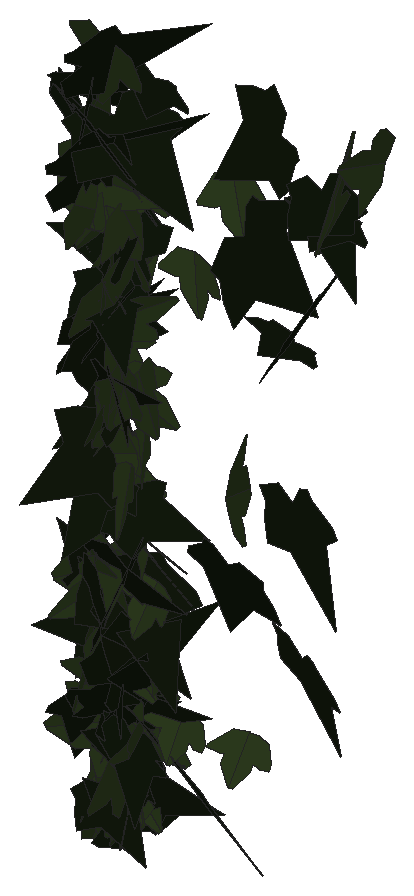
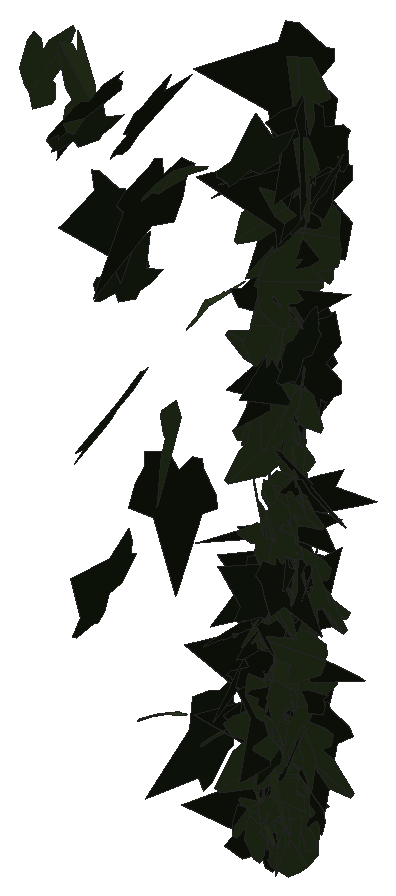
# SketchUp Ruby script. Lengths in inches.
U = 1.inch
M = Sketchup.active_model
def pt(a) = Geom::Point3d.new(a.map { |v| v * U })
def face(e, loops, mat)
  f = e.add_face(loops[0].map { |a| pt(a) })
  loops[1..].each { |l| e.add_face(l.map { |a| pt(a) }).erase! }
  f.material = f.back_material = mat if mat
  f
end
# faces: each face lists its corners as indices into pts; further lists are holes
def faces(e, pts, list, mat = nil) = list.each { |f| face(e, (f[0].is_a?(Array) ? f : [f]).map { |l| l.map { |i| pts[i] } }, mat) }
# xy, xz, yz: faces in a plane at the given z, y or x. An outline is a flat list of corners, or four numbers for a rectangle; further outlines are holes
def ring(l) = l.size == 4 ? [[l[0], l[1]], [l[2], l[1]], [l[2], l[3]], [l[0], l[3]]] : l.each_slice(2).to_a
def flat(e, list, mat, &to3) = list.each { |f| face(e, (f[0].is_a?(Array) ? f : [f]).map { |l| ring(l).map { |u, v| to3.(u, v) } }, mat) }
def xy(e, z, list, mat = nil) = flat(e, list, mat) { |x, y| [x, y, z] }
def xz(e, y, list, mat = nil) = flat(e, list, mat) { |x, z| [x, y, z] }
def yz(e, x, list, mat = nil) = flat(e, list, mat) { |y, z| [x, y, z] }
def lines(e, pts, list) = list.each { |a, b| e.add_line(pt(pts[a]), pt(pts[b])) }
# prism: a flat outline (further loops are holes) pulled along v
def prism(e, loops, v, mat = nil)
  f = face(e, loops, mat); d = Geom::Vector3d.new(v.map { |x| x * U })
  f.pushpull(f.normal.samedirection?(d) ? d.length : -d.length)
end
def box(e, o, s, mat = nil) = prism(e, [[o, [o[0] + s[0], o[1], o[2]], [o[0] + s[0], o[1] + s[1], o[2]], [o[0], o[1] + s[1], o[2]]]], [0, 0, s[2]], mat)
def at(x, y, z, deg = 0) = Geom::Transformation.translation(pt([x, y, z])) * Geom::Transformation.rotation(ORIGIN, Z_AXIS, deg.degrees)
def axes(o, x, y, z) = Geom::Transformation.new([*x, 0, *y, 0, *z, 0, *pt(o).to_a, 1])
def part(name) = M.definitions.add(name)
# library, detail: a bought-in or finely detailed component or shape, given as its bounding box
def library(name, o, s) = part(name).tap { |d| box(d.entities, o, s) }
def detail(e, o, s) = box(e.add_group.entities, o, s)
def put(e, d, t, mat = nil) = e.add_instance(d, t).tap { |i| i.material = mat if mat }
def group(e, t, mat = nil) = e.add_group.tap { |g| g.transformation = t; g.material = mat if mat }.entities
root = M.entities
M.materials.add("efeu1").color = [18, 25, 13]
M.materials.add("efeu2").color = [43, 57, 29]
c1 = part("ivyleaf_10")
p = [[0,0.5,-0.03],[-0.0625,2.02,-0.43],[-0.19,2.01,-0.46],[-0.54,1.05,-0.29],[-0.52,0.625,-0.18],[-0.83,0.76,-0.28],
  [-1.16,0.64,-0.33],[-1.15,0.33,-0.24],[-0.77,-0.39,0.02],[-0.3,-0.51,0.16],[0.04,-0.48,0.23],[-0.02,2.01,-0.4375],
  [-0.06,2.01,-0.43],[0.04,-0.49,0.23],[0.67,-0.49,0.14],[1.38,0.36,-0.2],[1.375,0.51,-0.24],[0.81,0.65,-0.19],
  [0.62,0.59,-0.15],[0.6,1.09,-0.28],[0.5,1.23,-0.31]]
faces(c1.entities,p,[[0,1,2,3,4,5,6,7,8,9,10],[11,12,0,13,14,15,16,17,18,19,20]],"efeu2")
c2 = part("ivyleaf_9")
p = [[1.54,2.16,1.25],[1.36,2.04,1.19],[-0.21,0.99,0.68],[-0.71,1.11,0.82],[-0.85,0.86,0.67],[-0.8,0.17,0.21],
  [-0.9,-0.01,0.1],[-0.67,-0.16,-0.02],[-0.08,-0.08,-0.05],[-0.03,-0.6,-0.4],[0.65,-0.88,-0.66],[0.83,-0.6,-0.49],
  [1.29,-0.42,-0.43],[1.8125,-0.07,-0.26],[1.21,0.44,0.15]]
faces(c2.entities,p,[[0,1,2,3,4,5,6,7,8,9,10,11,12,13,14]],"efeu1")
put(root,c1,axes([585.83,126.8,191.39],[0.53588,-0.21194,-0.8665],[-0.80039,0.33208,-0.57622],[0.39386,0.96318,0.008]))
put(root,c1,axes([585.97,126.76,206.64],[-0.97546,0.08442,0.38421],[-0.38156,0.04674,-0.97903],[-0.09566,-1.04736,-0.01272]))
put(root,c1,axes([585.76,127.4375,190.76],[0.22117,0.36477,-0.87026],[-0.59752,-0.63767,-0.41913],[-0.73033,0.63218,0.07937]))
put(root,c2,axes([585.8,126.18,206.35],[0.1962,0.8705,-0.7375],[0.14249,0.72377,0.8922],[1.13197,-0.24198,0.01552]))
put(root,c2,axes([585.68,127.14,191.08],[0.52201,-0.39717,0.77495],[0.6744,-0.3872,-0.65272],[0.55089,0.85036,0.06474]))
put(root,c2,axes([585.32,126.58,204.45],[1.26759,-0.16301,-0.50833],[-0.49862,0.10623,-1.27744],[0.19066,1.36158,0.0388]))
put(root,c2,axes([586.25,127.48,186.12],[0.08288,-0.84438,0.23188],[0.09411,-0.22298,-0.8456],[0.87057,0.1045,0.06934]))
put(root,c1,axes([586.25,127.21,193.9],[0.60781,-0.3979,0.23932],[0.19688,-0.13618,-0.72645],[0.42052,0.63888,-0.00579]))
put(root,c2,axes([590.04,126.7,192.86],[0.72145,0.31331,-0.76378],[-0.73389,-0.2211,-0.78392],[-0.37805,1.02712,0.06424]))
put(root,c2,axes([585.72,127.19,199.44],[0.00525,-0.77499,-0.26252],[0.01443,0.26258,-0.77485],[0.81812,0.00034,0.01535]))
put(root,c2,axes([586.1,127.62,185.38],[0.5714,-0.79133,-0.15741],[0.10342,-0.11947,0.97597],[-0.80018,-0.58053,0.01373]))
put(root,c2,axes([584.45,127.69,203.85],[0.19177,-0.77719,0.6517],[0.16789,-0.62977,-0.80044],[1.00027,0.2547,0.00941]))
put(root,c1,axes([585.67,127.17,188.01],[-0.73952,-0.35537,-0.0641],[-0.05305,-0.03758,0.8204],[-0.35719,0.74134,0.01087]))
put(root,c2,axes([585.59,127.45,193.39],[-0.59969,-0.49951,0.03874],[-0.02928,-0.02537,-0.78047],[0.50015,-0.60041,0.00076]))
put(root,c2,axes([585.74,127.01,184.65],[-0.2181,-0.29266,-0.67092],[0.47467,0.47636,-0.3621],[0.5572,-0.52036,0.04586]))
put(root,c1,axes([585.95,126.73,199.6],[-0.18116,-0.87389,-0.5283],[0.13264,0.51186,-0.89219],[1.01252,-0.22341,0.02236]))
put(root,c2,axes([585.31,127.78,194.21],[-0.59416,-0.54054,0.56045],[-0.38707,-0.40667,-0.80257],[0.67562,-0.70834,0.03308]))
put(root,c2,axes([585.73,127.15,186.94],[0.8681,0.5207,0.17599],[-0.15252,-0.08785,1.01228],[0.52805,-0.88139,0.00307]))
put(root,c2,axes([585.875,127.08,202.96],[0.24927,-0.25277,0.76845],[-0.58189,0.50257,0.35407],[-0.56197,-0.63251,-0.02576]))
put(root,c2,axes([585.68,127.51,196.34],[0.26604,-0.07043,-0.74306],[0.7081,-0.22562,0.27491],[-0.23601,-0.75632,-0.01281]))
put(root,c2,axes([585.64,127.28,190.48],[0.40618,-0.07857,0.7094],[-0.68976,0.1666,0.41338],[-0.18346,-0.8003,0.01641]))
put(root,c2,axes([585.38,127.25,196.36],[0.28354,-0.28326,0.65236],[0.60154,-0.27915,-0.38266],[0.37942,0.65425,0.11917]))
put(root,c1,axes([586.39,127.03,185.82],[0.12881,-1.16578,-0.32263],[0.12747,0.33573,-1.16222],[1.20286,0.08926,0.15772]))
put(root,c1,axes([586.01,127.07,196.53],[-0.72562,0.02431,0.27132],[-0.27156,-0.00338,-0.72594],[-0.02159,-0.77469,0.01168]))
put(root,c2,axes([585.23,126.3,202.9],[0.22606,1.05829,-0.73534],[0.08914,0.73194,1.0808],[1.2856,-0.23685,0.05436]))
put(root,c2,axes([585.64,127.29,189.57],[0.0896,0.87466,0.70671],[-0.07755,-0.70246,0.87923],[1.12181,-0.11842,0.00433]))
put(root,c1,axes([585.53,126.99,191.18],[-0.88666,0.21945,0.46734],[-0.45458,0.10852,-0.91341],[-0.24479,-0.99639,0.00345]))
put(root,c1,axes([586.01,127.17,197.09],[-0.62727,0.01494,0.45907],[-0.45909,-0.04439,-0.62586],[0.01418,-0.77605,0.04464]))
put(root,c2,axes([585.42,126.95,191.3125],[0.67678,-0.43776,-0.65378],[-0.55675,0.3429,-0.80594],[0.55596,0.87629,-0.01123]))
put(root,c2,axes([585.29,127.13,187.16],[0.25446,0.66269,-0.48536],[-0.16703,-0.45575,-0.70983],[-0.80425,0.30432,-0.00614]))
put(root,c2,axes([591.52,127.5625,194.73],[0.52714,-1.01866,0.01643],[0.00752,-0.01461,-1.14698],[1.01877,0.52719,-0.00003]))
put(root,c1,axes([585.21,126.77,201.78],[-0.12539,-0.48745,-0.72412],[0.24432,0.68272,-0.50188],[0.83802,-0.27198,0.03798]))
put(root,c2,axes([585.86,127.37,204.24],[0.33074,-1.05423,-0.43486],[0.41693,0.53322,-0.97558],[1.06145,0.11905,0.5187]))
put(root,c2,axes([588.22,127.22,185.86],[1.02842,-0.44574,-0.06664],[-0.0621,0.02431,-1.12086],[0.4464,1.03029,-0.00239]))
put(root,c1,axes([585.85,127.1875,188.89],[0.54081,0.29658,0.61881],[0.55533,0.27369,-0.61649],[-0.40311,0.77492,-0.0191]))
put(root,c1,axes([593.01,127.03,203.67],[0.62587,-0.96913,0.5274],[-0.28236,0.44547,1.15365],[-1.0666,-0.68661,0.00407]))
put(root,c1,axes([584.82,128.01,188.22],[-0.02958,0.51375,-0.97381],[0.08461,-0.97022,-0.51442],[-1.09776,-0.08863,-0.01341]))
put(root,c1,axes([584.8,127.11,202.35],[0.0716,-0.05686,1.17592],[1.06714,0.50069,-0.04077],[-0.49722,1.06641,0.08184]))
put(root,c1,axes([585.37,127.3,186.43],[0.44016,-0.14131,-0.89437],[-0.85731,0.25494,-0.4622],[0.29134,0.96366,-0.00887]))
put(root,c1,axes([585.79,127.25,183.84],[0.86466,-0.04091,0.48702],[-0.48644,0.02381,0.86562],[-0.04733,-0.99209,0.00069]))
put(root,c2,axes([585.25,126.47,197.9],[0.32694,0.4269,1.01324],[0.61647,0.80412,-0.53772],[-0.91041,0.6978,-0.00024]))
put(root,c2,axes([584.91,126.92,205.48],[0.59751,0.57819,0.05721],[0.04033,0.04058,-0.83146],[-0.57962,0.59887,0.00111]))
put(root,c1,axes([585.82,127.11,199.95],[0.25578,-0.56509,-0.49461],[-0.01825,0.51768,-0.60089],[0.75076,0.20511,0.1539]))
put(root,c2,axes([585.49,127.79,188.74],[-0.27034,-0.03197,-0.89567],[0.88746,-0.1402,-0.26286],[-0.12516,-0.92501,0.0708]))
put(root,c2,axes([586,126.86,199.89],[-0.65134,0.48148,-0.38102],[-0.32151,0.20578,0.80965],[0.5231,0.726,0.0232]))
put(root,c1,axes([586.51,127.96,190.28],[-0.43545,-0.3158,0.48137],[0.30919,-0.63741,-0.13847],[0.48564,0.12266,0.51978]))
put(root,c2,axes([585.44,126.8125,205.26],[-0.15113,0.12633,-1.05155],[-0.94101,0.47141,0.19188],[0.48601,0.95203,0.04453]))
put(root,c2,axes([585.625,126.68,198.32],[0.00754,0.13958,-1.05071],[-0.47909,0.93773,0.12114],[0.94549,0.47405,0.06976]))
put(root,c2,axes([586.34,126.72,188.29],[0.08703,0.09456,1.15071],[0.90737,0.70799,-0.12681],[-0.71397,0.9113,-0.02088]))
put(root,c1,axes([585.91,127.8,184.3],[0.45465,-0.425,0.3532],[0.25259,-0.24698,-0.62232],[0.4915,0.52006,-0.0069]))
put(root,c1,axes([585.9,127.77,187.81],[0.17584,-0.19445,-0.82175],[0.709,-0.42194,0.25156],[-0.45869,-0.72674,0.07382]))
put(root,c2,axes([585.78,127.89,189.2],[-0.23962,-0.32089,-0.76814],[-0.47974,-0.60003,0.40031],[-0.68034,0.53612,-0.01174]))
put(root,c1,axes([586.13,128.01,188.53],[0.01931,-0.60249,0.55135],[0.0076,-0.55134,-0.60276],[0.81666,0.01938,-0.00743]))
put(root,c2,axes([585.96,127.92,190.6],[0.14104,-1.25014,-0.21359],[0.2943,0.2413,-1.218],[1.23363,0.08536,0.31499]))
put(root,c1,axes([585.23,127.54,195.44],[0.26871,-0.69004,-0.15428],[-0.05087,0.14575,-0.74049],[0.70524,0.27343,0.00537]))
put(root,c1,axes([585.75,127.67,193.63],[0.632,-0.47735,-0.00847],[-0.00715,0.00459,-0.79202],[0.47738,0.63205,-0.00065]))
put(root,c2,axes([586.125,127.95,183.26],[0.29169,0.11087,0.77873],[-0.72264,-0.29025,0.31201],[0.31066,-0.77927,-0.00542]))
put(root,c2,axes([591.91,126.73,200.08],[-0.47279,0.84163,-0.58854],[-0.33232,0.48768,0.96436],[0.97174,0.57627,0.04345]))
put(root,c1,axes([585.2,127.5,183.17],[-0.09684,-0.67219,0.2522],[0.03481,0.24979,0.67913],[-0.7171,0.1029,-0.00109]))
put(root,c2,axes([585.32,128.22,185.88],[0.51336,-0.56939,-0.46718],[0.41143,-0.25064,0.75756],[-0.61089,-0.64728,0.11762]))
put(root,c2,axes([592.27,127.78,204.1],[0.27473,-0.90215,-0.28451],[-0.07801,0.27365,-0.94304],[0.94273,0.28555,0.00487]))
put(root,c1,axes([585.87,127.27,196.78],[0.12099,-0.14786,-0.78458],[-0.49273,0.61056,-0.19105],[0.62821,0.50736,0.00126]))
put(root,c1,axes([585.49,127.59,184.32],[-0.60782,0.29266,-0.11803],[0.11122,-0.04105,-0.67452],[-0.29531,-0.61782,-0.0111]))
put(root,c2,axes([590.83,128.33,199.05],[-0.47179,-0.40595,0.44745],[0.27112,-0.64961,-0.30349],[0.53991,-0.02853,0.5434]))
put(root,c2,axes([592.24,128.37,203.25],[-0.3902,-0.57439,0.39897],[0.31429,-0.55216,-0.48755],[0.62477,-0.08097,0.49444]))
put(root,c2,axes([586.15,127.48,192.89],[0.47741,-0.37824,-0.45674],[0.24337,0.65966,-0.29192],[0.54079,0.03705,0.53458]))
put(root,c1,axes([585.37,127.38,192.36],[0.17489,-0.38565,-0.6066],[-0.16915,0.58469,-0.42048],[0.69862,0.2381,0.05005]))
put(root,c1,axes([586.34,127.68,196.52],[0.08422,-0.85682,-0.20288],[0.27409,0.21919,-0.81193],[0.83677,0.01444,0.28637]))
put(root,c1,axes([586.02,128.21,184.18],[0.01978,-0.5715,0.51697],[0.03905,-0.51573,-0.57163],[0.76964,0.04085,0.01572]))
put(root,c1,axes([589.1,128.13,203.05],[-0.35159,-0.68172,0.18485],[0.5573,-0.3946,-0.39527],[0.43397,-0.04557,0.65736]))
put(root,c1,axes([585.75,127.71,194.26],[0.26305,-0.07968,-0.74976],[-0.71934,0.21142,-0.27484],[0.22593,0.76592,-0.00213]))
put(root,c1,axes([585.6,127.74,201.66],[0.23057,0.7483,-0.01298],[-0.00333,-0.01255,-0.78301],[-0.7484,0.23059,-0.00051]))
put(root,c2,axes([585.97,127.59,186.94],[0.4553,-0.04204,0.62477],[0.62523,-0.01205,-0.45645],[0.03451,0.77297,0.02687]))
put(root,c1,axes([585.89,127.59,201.39],[0.08698,-0.84374,-0.3788],[0.28376,0.38647,-0.79566],[0.88027,-0.04121,0.29392]))
put(root,c2,axes([585.98,127.51,190.23],[0.58247,-0.72842,-0.76211],[-0.40552,0.64889,-0.93014],[0.97311,0.70641,0.06855]))
put(root,c1,axes([585.83,127.65,202.88],[0.52987,0.21475,0.65238],[0.58499,0.2906,-0.5708],[-0.35986,0.78861,0.03269]))
put(root,c1,axes([585.75,127.59,198.24],[-0.23336,-0.42295,0.66694],[0.52275,0.43856,0.46103],[-0.59197,0.55401,0.14421]))
put(root,c1,axes([585.4,127.77,187.52],[-0.01596,-0.68847,-0.15062],[-0.01089,0.15088,-0.68851],[0.70467,-0.01326,-0.01405]))
put(root,c1,axes([587.2,128.3125,186.6],[-0.53665,-0.32172,0.29703],[0.30418,-0.61188,-0.11316],[0.31497,0.04277,0.61538]))
put(root,c1,axes([585.82,127.63,188.06],[-0.58867,0.30011,0.3317],[-0.3214,0.09754,-0.65864],[-0.31111,-0.66861,0.0528]))
put(root,c1,axes([585.25,128.15,194.36],[0.11954,0.49335,-0.53767],[-0.273,-0.47503,-0.49657],[-0.67672,0.27878,0.10535]))
put(root,c2,axes([586.05,128.1,199.99],[-0.26852,0.01899,0.83145],[-0.83083,-0.04537,-0.26728],[0.03736,-0.87256,0.03199]))
put(root,c1,axes([584.89,127.96,197.875],[-0.19863,0.66982,-0.30674],[0.0686,-0.2995,-0.69843],[-0.73352,-0.20939,0.01774]))
put(root,c2,axes([584.53,128.27,199.1875],[0.2537,-0.48451,0.60376],[0.31602,-0.51518,-0.54622],[0.70669,0.40432,0.02751]))
put(root,c2,axes([585.62,127.02,197.95],[-0.31859,0.5893,-0.74967],[-0.40495,0.63197,0.66888],[0.8633,0.51391,0.0371]))
put(root,c1,axes([585.85,128.06,183.95],[0.43401,-0.46796,-0.35633],[0.26174,-0.24292,0.63782],[-0.52674,-0.50629,0.02333]))
put(root,c1,axes([585.14,128.67,201.41],[0.03073,-0.38095,0.97527],[0.18655,-0.95809,-0.38012],[1.03028,0.18484,0.03973]))
put(root,c2,axes([586.125,128.43,189.09],[-0.54233,-0.5012,0.28586],[-0.20928,-0.19473,-0.73846],[0.5377,-0.58131,0.00091]))
put(root,c2,axes([590.14,127.35,202.24],[0.38346,-0.5039,-1.08095],[-0.57521,0.91652,-0.6313],[1.04475,0.68955,0.04917]))
put(root,c2,axes([585.25,128.04,195.54],[-0.79186,0.22291,0.03186],[-0.02904,0.01443,-0.82262],[-0.2233,-0.79237,-0.00602]))
put(root,c1,axes([585.52,127.99,194.4],[0.70987,-0.18038,-0.11133],[-0.104,0.04266,-0.73226],[0.18471,0.71728,0.01555]))
put(root,c2,axes([591.08,128.45,189.67],[0.46264,-0.83971,0.54607],[0.29292,-0.46178,-0.95827],[0.95786,0.54679,0.0293]))
put(root,c1,axes([586.1,128.43,184.55],[-0.36602,-0.41306,0.42726],[0.30951,-0.56087,-0.27708],[0.50732,0.04416,0.4773]))
put(root,c1,axes([585.0625,127.67,204.92],[0.59002,-0.34944,-0.56806],[-0.30326,0.53494,-0.64405],[0.59399,0.62021,0.23545]))
put(root,c2,axes([589.92,128.87,204.54],[-0.25518,-0.52996,0.88702],[-0.22368,-0.86368,-0.58036],[1.00878,-0.32557,0.09569]))
put(root,c1,axes([589.18,128.49,186.55],[-0.61575,-0.25747,0.14371],[0.23105,-0.62804,-0.13523],[0.1832,-0.07333,0.65357]))
put(root,c1,axes([585.23,127.95,197.47],[-0.71082,-0.33234,-0.28939],[0.31561,-0.00063,-0.7745],[0.30755,-0.76747,0.12595]))
put(root,c1,axes([585.625,127.74,186.76],[-0.81796,-0.29092,-0.79368],[0.76357,0.21954,-0.8674],[0.36267,-1.11839,0.03619]))
put(root,c1,axes([585.32,128.32,185.28],[0.23197,0.37424,-0.51833],[-0.31363,-0.41387,-0.43919],[-0.5571,0.38883,0.03142]))
put(root,c1,axes([585.67,127.51,183.74],[-0.11417,0.1404,0.75451],[-0.49889,0.56608,-0.18083],[-0.58319,-0.51174,0.00698]))
put(root,c1,axes([589.74,127.34,194.52],[-0.22448,0.35407,1.05328],[-0.69989,0.78957,-0.41458],[-0.86309,-0.73237,0.06225]))
put(root,c2,axes([585.38,128.22,192.29],[-0.42507,0.5155,-0.43865],[0.20578,-0.39504,-0.66365],[-0.64483,-0.46587,0.07737]))
put(root,c1,axes([585.49,128.67,200.0625],[0.16602,0.37112,-0.87286],[-0.3919,-0.78011,-0.40623],[-0.86373,0.42529,0.01654]))
put(root,c2,axes([585,128.13,188.52],[-0.06887,-0.56477,-0.52412],[0.35023,0.44576,-0.52635],[0.6863,-0.28415,0.21601]))
put(root,c1,axes([593.27,128.8,204.92],[-0.05449,-0.30842,-0.89808],[-0.13612,-0.88773,0.31313],[-0.93976,0.14646,0.00672]))
put(root,c1,axes([585.45,128.1,185.91],[0.19311,-0.71958,-0.14347],[-0.05618,0.13342,-0.7448],[0.73159,0.20019,-0.01932]))
put(root,c1,axes([585.83,128.04,191.46],[0.55869,-0.26813,-0.49498],[-0.43987,0.22727,-0.6196],[0.35131,0.71098,0.01138]))
put(root,c1,axes([585.8,128.04,184.34],[0.45275,0.208,0.45075],[0.42159,0.161,-0.49775],[-0.2621,0.61825,-0.02202]))
put(root,c2,axes([586.03,127.89,184.48],[0.30739,0.15123,-0.76841],[0.52008,0.57775,0.32176],[0.58552,-0.59257,0.1176]))
put(root,c2,axes([585.33,128.28,186.82],[0.55675,-0.48775,0.18997],[0.15251,-0.11415,-0.74005],[0.50073,0.57709,0.01417]))
put(root,c1,axes([585.65,127.91,196.125],[-0.55772,-0.36995,-0.62401],[0.56705,0.26859,-0.66605],[0.45245,-0.79265,0.06555]))
put(root,c1,axes([587.36,128.63,199.91],[-0.34716,-0.55975,0.44285],[0.5886,-0.50306,-0.17444],[0.40371,0.25211,0.63515]))
put(root,c1,axes([585.95,128.2,187.2],[-0.64158,0.07204,-0.24303],[0.22093,-0.16533,-0.63224],[-0.12427,-0.66585,0.13069]))
put(root,c1,axes([585.35,128.4,187.03],[0.25821,0.58881,-0.42977],[-0.28794,-0.33648,-0.63399],[-0.66969,0.37169,0.10688]))
put(root,c1,axes([585.77,128,189.26],[-0.46887,0.4826,0.20589],[-0.18737,0.1039,-0.67025],[-0.49009,-0.50143,0.05928]))
put(root,c1,axes([585.97,127.67,184.2],[-0.03763,0.15287,-0.71125],[-0.15748,0.69361,0.15741],[0.71025,0.16189,-0.00278]))
put(root,c1,axes([585.7,128.28,190.66],[0.02941,0.6795,-0.21705],[-0.01191,-0.21673,-0.68013],[-0.71322,0.03164,0.00241]))
put(root,c1,axes([585.57,128.2,193.18],[0.68032,0.23677,0.1429],[0.12869,0.06484,-0.72011],[-0.24478,0.69214,0.01857]))
put(root,c2,axes([585.86,128.125,191.59],[0.73235,-0.30916,0.02784],[0.02633,-0.00923,-0.79493],[0.30929,0.73282,0.00173]))
put(root,c1,axes([585.63,128.15,199.59],[-0.62942,0.41741,-0.14917],[0.1173,-0.09298,-0.75515],[-0.42746,-0.64014,0.01242]))
put(root,c2,axes([585.95,127.45,187.18],[0.12581,0.71807,0.61599],[0.10749,0.60654,-0.72901],[-0.93995,0.16547,-0.00092]))
put(root,c1,axes([585.01,128.61,189.05],[-0.17705,0.52894,-0.56856],[-0.25578,-0.59033,-0.46955],[-0.73323,0.07821,0.30109]))
put(root,c2,axes([585.84,128.84,204.82],[-0.21913,-0.65162,0.51965],[0.40862,-0.5523,-0.52025],[0.72642,0.11411,0.44941]))
put(root,c1,axes([585.75,128.49,194.23],[0.57329,-0.36428,0.36996],[0.31753,-0.19005,-0.67918],[0.41079,0.65529,0.00868]))
put(root,c2,axes([585.5,128.47,191.59],[0.34763,-0.50723,0.51828],[0.48741,-0.26216,-0.58348],[0.53697,0.56634,0.1941]))
put(root,c1,axes([584.37,128.03,189.85],[0.18506,0.04422,-0.69226],[0.66796,0.18189,0.19018],[0.1871,-0.6931,0.00574]))
